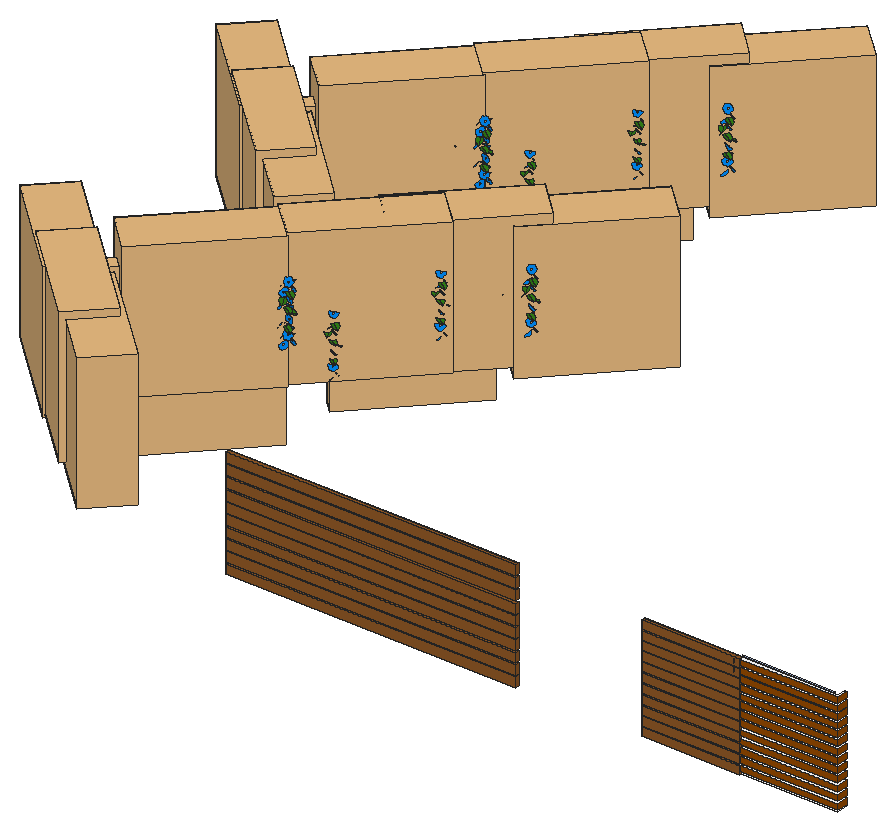
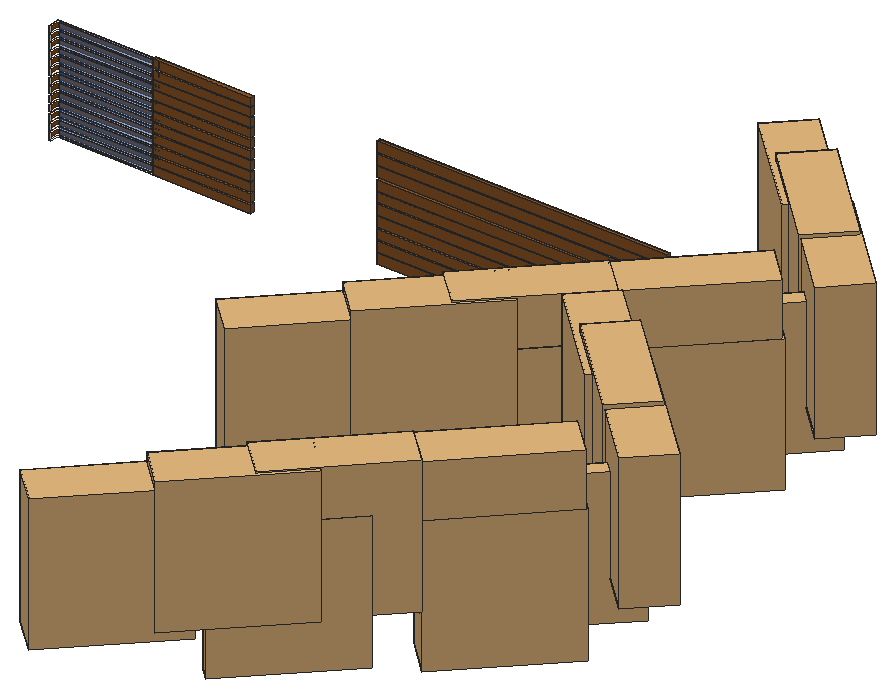
# SketchUp Ruby script. Lengths in inches.
U = 1.inch
M = Sketchup.active_model
def pt(a) = Geom::Point3d.new(a.map { |v| v * U })
def face(e, loops, mat)
  f = e.add_face(loops[0].map { |a| pt(a) })
  loops[1..].each { |l| e.add_face(l.map { |a| pt(a) }).erase! }
  f.material = f.back_material = mat if mat
  f
end
# faces: each face lists its corners as indices into pts; further lists are holes
def faces(e, pts, list, mat = nil) = list.each { |f| face(e, (f[0].is_a?(Array) ? f : [f]).map { |l| l.map { |i| pts[i] } }, mat) }
# xy, xz, yz: faces in a plane at the given z, y or x. An outline is a flat list of corners, or four numbers for a rectangle; further outlines are holes
def ring(l) = l.size == 4 ? [[l[0], l[1]], [l[2], l[1]], [l[2], l[3]], [l[0], l[3]]] : l.each_slice(2).to_a
def flat(e, list, mat, &to3) = list.each { |f| face(e, (f[0].is_a?(Array) ? f : [f]).map { |l| ring(l).map { |u, v| to3.(u, v) } }, mat) }
def xy(e, z, list, mat = nil) = flat(e, list, mat) { |x, y| [x, y, z] }
def xz(e, y, list, mat = nil) = flat(e, list, mat) { |x, z| [x, y, z] }
def yz(e, x, list, mat = nil) = flat(e, list, mat) { |y, z| [x, y, z] }
def lines(e, pts, list) = list.each { |a, b| e.add_line(pt(pts[a]), pt(pts[b])) }
# prism: a flat outline (further loops are holes) pulled along v
def prism(e, loops, v, mat = nil)
  f = face(e, loops, mat); d = Geom::Vector3d.new(v.map { |x| x * U })
  f.pushpull(f.normal.samedirection?(d) ? d.length : -d.length)
end
def box(e, o, s, mat = nil) = prism(e, [[o, [o[0] + s[0], o[1], o[2]], [o[0] + s[0], o[1] + s[1], o[2]], [o[0], o[1] + s[1], o[2]]]], [0, 0, s[2]], mat)
def at(x, y, z, deg = 0) = Geom::Transformation.translation(pt([x, y, z])) * Geom::Transformation.rotation(ORIGIN, Z_AXIS, deg.degrees)
def axes(o, x, y, z) = Geom::Transformation.new([*x, 0, *y, 0, *z, 0, *pt(o).to_a, 1])
def part(name) = M.definitions.add(name)
# library, detail: a bought-in or finely detailed component or shape, given as its bounding box
def library(name, o, s) = part(name).tap { |d| box(d.entities, o, s) }
def detail(e, o, s) = box(e.add_group.entities, o, s)
def put(e, d, t, mat = nil) = e.add_instance(d, t).tap { |i| i.material = mat if mat }
def group(e, t, mat = nil) = e.add_group.tap { |g| g.transformation = t; g.material = mat if mat }.entities
root = M.entities
M.materials.add("[Color C07]").color = [153, 76, 0]
M.materials.add("[Color M00]").color = [255, 255, 255]
M.materials.add("[Granite Tile]").color = [155, 148, 143]
M.materials.add("[Translucent Glass Blue]").color = [100, 149, 237]
M.materials["[Translucent Glass Blue]"].alpha = 0.5
M.materials.add("[Wood Floor Parquet]").color = [145, 89, 39]
M.materials.add("skp avat flo 1").color = [0, 129, 229]
M.materials.add("skp avat flo 2").color = [47, 120, 22]
c1 = part("Group\#24")
box(c1.entities,[0,-2.3125,0],[173.47,2.3125,5.79])
c2 = part("Group\#17")
box(c2.entities,[0,-2.125,0],[58.6875,4.9375,2.3125])
c3 = library("ruselia",[-5.83,-15.14,-32.53],[55.24,20.14,57.16])
c4 = part("Gruppe\#2")
xy(c4.entities,0,[[6.69,0,4.96,0.23,3.03,1.59,1.96,1.96,0.9,3.35,0.9,5.71,0,6.69,0.23,8.43,1.96,10,3.35,12.49,4.67,13.04,7.04,12.49,8.72,13.04,10.04,12.49,11.43,11.43,12.05,9.15,13.39,6.69,13.16,4.96,12.49,3.35,10.41,2.22,8.43,0.23]],"skp avat flo 1")
c5 = part("Gruppe\#12")
xy(c5.entities,0,[[1.18,0.5,1.36,0.52,1.52,0.59,1.67,0.7,1.77,0.84,1.84,1,1.87,1.18,1.84,1.36,1.77,1.52,1.67,1.67,1.52,1.77,1.36,1.84,1.18,1.87,1,1.84,0.84,1.77,0.7,1.67,0.59,1.52,0.52,1.36,0.5,1.18,0.52,1,0.59,0.84,0.7,0.7,0.84,0.59,1,0.52]])
c6 = part("f.st. wop plant 01 blüte")
put(c6.entities,c4,at(0,0,0))
put(c6.entities,c5,at(5.65,5.41,0.39))
c7 = part("Gruppe\#5")
xy(c7.entities,0.96,[[13.97,0.22,8.73,4.42,7.37,10.11,8.43,14.53,13.97,16.39]],"skp avat flo 2")
p = [[13.97,0.22,0.96],[13.97,16.39,0.96],[17.89,14.53,4.875],[18.64,10.11,5.625],[17.67,4.42,4.66]]
faces(c7.entities,p,[[0,1,2,3,4]],"skp avat flo 2")
c8 = part("f.st. wop plant 01 blatt")
put(c8.entities,c7,axes([0.99,0,4.74],[0.91566,0,-0.40195],[0,1,0],[0.40195,0,0.91566]))
c9 = part("Gruppe\#10")
put(c9.entities,c6,axes([4.61,0.45,57.14],[0.99373,-0.06775,-0.08889],[0.11172,0.62588,0.77188],[0.00335,-0.77697,0.62953]))
put(c9.entities,c6,axes([12.4,0.4,0.59],[0.70061,0.70799,-0.08889],[-0.40079,0.49353,0.77188],[0.59035,-0.50516,0.62953]))
put(c9.entities,c6,axes([24.4375,6.09,17.58],[-0.05734,0.99439,-0.08889],[-0.63495,0.03239,0.77188],[0.77043,0.1007,0.62953]))
put(c9.entities,c6,axes([1.11,8.09,13.25],[0.88983,-0.44754,-0.08889],[0.34553,0.53368,0.77188],[-0.298,-0.71756,0.62953]))
put(c9.entities,c6,axes([23.26,15,37.53],[-0.84836,0.52191,-0.08889],[-0.38985,-0.50222,0.77188],[0.35821,0.68948,0.62953]))
put(c9.entities,c6,axes([12.67,23.61,24.88],[-0.75852,-0.64555,-0.08889],[0.35717,-0.52596,0.77188],[-0.54504,0.55374,0.62953]))
put(c9.entities,c6,axes([20.43,22.9,81.42],[-0.98432,0.15238,-0.08889],[-0.16477,-0.61405,0.77188],[0.06303,0.77442,0.62953]))
put(c9.entities,c6,axes([1.76,2.9,29.21],[0.93833,-0.33412,-0.08889],[0.27691,0.5723,0.77188],[-0.20703,-0.74889,0.62953]))
put(c9.entities,c6,axes([13.59,0.5,77.09],[0.62412,0.77625,-0.08889],[-0.4494,0.44972,0.77188],[0.63915,-0.4418,0.62953]))
put(c9.entities,c6,axes([-1.26,15.51,69.79],[0.24265,-0.96603,-0.08889],[0.62977,0.08716,0.77188],[-0.73791,-0.24328,0.62953]))
put(c9.entities,c6,axes([22.04,17.92,65.46],[-0.95793,0.27287,-0.08889],[-0.2394,-0.58898,0.77188],[0.15827,0.76069,0.62953]))
put(c9.entities,c6,axes([9.51,23.35,52.81],[-0.55554,-0.82673,-0.08889],[0.48617,-0.40969,0.77188],[-0.67455,0.38559,0.62953]))
put(c9.entities,c6,axes([0.1875,18.97,41.86],[-0.02781,-0.99565,-0.08889],[0.62986,-0.08651,0.77188],[-0.77621,-0.03452,0.62953]))
put(c9.entities,c6,axes([24.98,7.4,94.08],[-0.15925,0.98323,-0.08889],[-0.63491,-0.03305,0.77188],[0.75599,0.17936,0.62953]))
put(c9.entities,c6,axes([21.5,21.98,4.93],[-0.96344,0.25275,-0.08889],[-0.22702,-0.59386,0.77188],[0.1423,0.76384,0.62953]))
put(c9.entities,c6,axes([1.57,6.98,89.75],[0.93112,-0.3537,-0.08889],[0.28884,0.56637,0.77188],[-0.22267,-0.74439,0.62953]))
put(c9.entities,c8,axes([9.37,32.32,90.95],[-0.51317,-0.65235,0],[0.5996,-0.47167,0.32697],[-0.25699,0.20216,0.76288]))
put(c9.entities,c8,axes([33.81,6.72,78.35],[-0.27992,0.78137,0],[-0.71819,-0.25729,0.32697],[0.30782,0.11027,0.76288]))
put(c9.entities,c8,axes([-9.46,14.86,61.47],[0.53029,-0.63851,0],[0.58688,0.4874,0.32697],[-0.25154,-0.2089,0.76288]))
put(c9.entities,c8,axes([21.49,-6.15,66.98],[0.2591,0.78852,0],[-0.72476,0.23815,0.32697],[0.31063,-0.10207,0.76288]))
put(c9.entities,c8,axes([32.03,5.27,54.38],[-0.36397,0.74594,0],[-0.68562,-0.33454,0.32697],[0.29386,0.14338,0.76288]))
put(c9.entities,c8,axes([30.63,20.6,49.31],[-0.77544,0.29596,0],[-0.27203,-0.71273,0.32697],[0.11659,0.30548,0.76288]))
put(c9.entities,c8,axes([32.03,5.27,27.16],[-0.36397,0.74594,0],[-0.68562,-0.33454,0.32697],[0.29386,0.14338,0.76288]))
put(c9.entities,c8,axes([17.4375,27.53,13.8125],[-0.76735,-0.23527,0.21148],[0.29408,-0.735,0.24937],[0.11659,0.30548,0.76288]))
put(c9.entities,c8,axes([-9.46,14.86,34.24],[0.53029,-0.63851,0],[0.58688,0.4874,0.32697],[-0.25154,-0.2089,0.76288]))
c10 = part("Gruppe\#9")
put(c10.entities,c6,axes([2.2,1.62,57.61],[0.97169,-0.0623,-0.22792],[0.22172,0.57378,0.78843],[0.08166,-0.81664,0.57134]))
put(c10.entities,c6,axes([-1.48,7.53,1.27],[0.68093,0.71536,-0.15682],[-0.22028,0.40428,0.88771],[0.69843,-0.56993,0.43287]))
put(c10.entities,c6,axes([13.97,11.34,15.86],[-0.0542,0.99797,0.03349],[-0.45869,-0.05467,0.88691],[0.88694,0.03271,0.46072]))
put(c10.entities,c6,axes([-9.71,13.74,16.77],[0.84218,-0.4326,-0.32186],[0.5102,0.4462,0.73526],[-0.17446,-0.78343,0.59649]))
put(c10.entities,c6,axes([17.17,17.99,36.46],[-0.83727,0.52624,0.14846],[-0.23006,-0.58536,0.77745],[0.49603,0.61679,0.61117]))
put(c10.entities,c6,axes([4.35,27.92,27.32],[-0.77345,-0.63385,0.00301],[0.4998,-0.60694,0.61792],[-0.38984,0.47943,0.78623]))
put(c10.entities,c6,axes([20.43,22.9,81.42],[-0.98432,0.15238,-0.08889],[-0.16477,-0.61405,0.77188],[0.06303,0.77442,0.62953]))
put(c10.entities,c6,axes([-5.84,6.82,31.58],[0.89192,-0.31974,-0.31975],[0.44391,0.4844,0.75386],[-0.08616,-0.81432,0.57398]))
put(c10.entities,c6,axes([13.59,0.5,77.09],[0.62412,0.77625,-0.08889],[-0.4494,0.44972,0.77188],[0.63915,-0.4418,0.62953]))
put(c10.entities,c6,axes([-1.26,15.51,69.79],[0.24265,-0.96603,-0.08889],[0.62977,0.08716,0.77188],[-0.73791,-0.24328,0.62953]))
put(c10.entities,c6,axes([20.77,18.5,64.59],[-0.95848,0.27864,0.06062],[-0.13765,-0.63827,0.75741],[0.24973,0.71762,0.65012]))
put(c10.entities,c6,axes([6.6875,24.75,54.15],[-0.57029,-0.8188,-0.06577],[0.58283,-0.45976,0.67002],[-0.57885,0.34377,0.73942]))
put(c10.entities,c6,axes([-4.08,21.11,44.3125],[-0.04911,-0.98765,-0.14878],[0.72825,-0.13735,0.67141],[-0.68355,-0.07538,0.726]))
put(c10.entities,c6,axes([24.98,7.4,94.08],[-0.15925,0.98323,-0.08889],[-0.63491,-0.03305,0.77188],[0.75599,0.17936,0.62953]))
put(c10.entities,c6,axes([8.77,28.52,5.9],[-0.95532,0.25842,0.14346],[-0.07274,-0.676,0.7333],[0.28648,0.6901,0.6646]))
put(c10.entities,c6,axes([1.57,6.98,89.75],[0.93112,-0.3537,-0.08889],[0.28884,0.56637,0.77188],[-0.22267,-0.74439,0.62953]))
put(c10.entities,c8,axes([9.37,32.32,90.95],[-0.51317,-0.65235,0],[0.5996,-0.47167,0.32697],[-0.25699,0.20216,0.76288]))
put(c10.entities,c8,axes([33.81,6.72,78.35],[-0.27992,0.78137,0],[-0.71819,-0.25729,0.32697],[0.30782,0.11027,0.76288]))
put(c10.entities,c8,axes([-11.01,15.72,64.74],[0.51926,-0.63742,-0.11388],[0.63054,0.46456,0.27478],[-0.14729,-0.25842,0.77487]))
put(c10.entities,c8,axes([20.21,-5.625,64.6],[0.26417,0.78668,0.01588],[-0.67119,0.21655,0.43762],[0.41063,-0.15212,0.70508]))
put(c10.entities,c8,axes([29.04,6.59,51.45],[-0.35348,0.74452,0.09816],[-0.63785,-0.35493,0.39506],[0.39635,0.09281,0.72332]))
put(c10.entities,c8,axes([27.11,22.23,47.625],[-0.76537,0.29574,0.12508],[-0.23173,-0.73252,0.31403],[0.22228,0.25465,0.75805]))
put(c10.entities,c8,axes([23.375,9.49,23.48],[-0.34051,0.7404,0.15735],[-0.60881,-0.37042,0.42548],[0.44978,0.05914,0.69506]))
put(c10.entities,c8,axes([6.77,33.04,15.99],[-0.71083,-0.25923,0.3412],[0.32455,-0.75723,0.10082],[0.2798,0.21977,0.74988]))
put(c10.entities,c8,axes([-15.51,18.125,40.12],[0.50532,-0.63318,-0.18065],[0.65217,0.44994,0.24724],[-0.09068,-0.29247,0.77145]))
c11 = part("Gruppe\#11")
put(c11.entities,c6,axes([4.61,0.45,57.14],[0.99373,-0.06775,-0.08889],[0.11172,0.62588,0.77188],[0.00335,-0.77697,0.62953]))
put(c11.entities,c6,axes([12.4,0.4,0.59],[0.70061,0.70799,-0.08889],[-0.40079,0.49353,0.77188],[0.59035,-0.50516,0.62953]))
put(c11.entities,c6,axes([24.4375,6.09,17.58],[-0.05734,0.99439,-0.08889],[-0.63495,0.03239,0.77188],[0.77043,0.1007,0.62953]))
put(c11.entities,c6,axes([1.11,8.09,13.25],[0.88983,-0.44754,-0.08889],[0.34553,0.53368,0.77188],[-0.298,-0.71756,0.62953]))
put(c11.entities,c6,axes([23.26,15,37.53],[-0.84836,0.52191,-0.08889],[-0.38985,-0.50222,0.77188],[0.35821,0.68948,0.62953]))
put(c11.entities,c6,axes([12.67,23.61,24.88],[-0.75852,-0.64555,-0.08889],[0.35717,-0.52596,0.77188],[-0.54504,0.55374,0.62953]))
put(c11.entities,c6,axes([20.43,22.9,81.42],[-0.98432,0.15238,-0.08889],[-0.16477,-0.61405,0.77188],[0.06303,0.77442,0.62953]))
put(c11.entities,c6,axes([1.76,2.9,29.21],[0.93833,-0.33412,-0.08889],[0.27691,0.5723,0.77188],[-0.20703,-0.74889,0.62953]))
put(c11.entities,c6,axes([13.59,0.5,77.09],[0.62412,0.77625,-0.08889],[-0.4494,0.44972,0.77188],[0.63915,-0.4418,0.62953]))
put(c11.entities,c6,axes([-1.26,15.51,69.79],[0.24265,-0.96603,-0.08889],[0.62977,0.08716,0.77188],[-0.73791,-0.24328,0.62953]))
put(c11.entities,c6,axes([22.04,17.92,65.46],[-0.95793,0.27287,-0.08889],[-0.2394,-0.58898,0.77188],[0.15827,0.76069,0.62953]))
put(c11.entities,c6,axes([9.51,23.35,52.81],[-0.55554,-0.82673,-0.08889],[0.48617,-0.40969,0.77188],[-0.67455,0.38559,0.62953]))
put(c11.entities,c6,axes([0.1875,18.97,41.86],[-0.02781,-0.99565,-0.08889],[0.62986,-0.08651,0.77188],[-0.77621,-0.03452,0.62953]))
put(c11.entities,c6,axes([24.98,7.4,94.08],[-0.15925,0.98323,-0.08889],[-0.63491,-0.03305,0.77188],[0.75599,0.17936,0.62953]))
put(c11.entities,c6,axes([21.5,21.98,4.93],[-0.96344,0.25275,-0.08889],[-0.22702,-0.59386,0.77188],[0.1423,0.76384,0.62953]))
put(c11.entities,c6,axes([1.57,6.98,89.75],[0.93112,-0.3537,-0.08889],[0.28884,0.56637,0.77188],[-0.22267,-0.74439,0.62953]))
put(c11.entities,c8,axes([9.37,32.32,90.95],[-0.51317,-0.65235,0],[0.5996,-0.47167,0.32697],[-0.25699,0.20216,0.76288]))
put(c11.entities,c8,axes([33.81,6.72,78.35],[-0.27992,0.78137,0],[-0.71819,-0.25729,0.32697],[0.30782,0.11027,0.76288]))
put(c11.entities,c8,axes([-9.46,14.86,61.47],[0.53029,-0.63851,0],[0.58688,0.4874,0.32697],[-0.25154,-0.2089,0.76288]))
put(c11.entities,c8,axes([21.49,-6.15,66.98],[0.2591,0.78852,0],[-0.72476,0.23815,0.32697],[0.31063,-0.10207,0.76288]))
put(c11.entities,c8,axes([32.03,5.27,54.38],[-0.36397,0.74594,0],[-0.68562,-0.33454,0.32697],[0.29386,0.14338,0.76288]))
put(c11.entities,c8,axes([30.63,20.6,49.31],[-0.77544,0.29596,0],[-0.27203,-0.71273,0.32697],[0.11659,0.30548,0.76288]))
put(c11.entities,c8,axes([32.03,5.27,27.16],[-0.36397,0.74594,0],[-0.68562,-0.33454,0.32697],[0.29386,0.14338,0.76288]))
put(c11.entities,c8,axes([17.4375,27.53,13.8125],[-0.76735,-0.23527,0.21148],[0.29408,-0.735,0.24937],[0.11659,0.30548,0.76288]))
put(c11.entities,c8,axes([-9.46,14.86,34.24],[0.53029,-0.63851,0],[0.58688,0.4874,0.32697],[-0.25154,-0.2089,0.76288]))
c12 = part("Gruppe\#8")
put(c12.entities,c6,axes([2.26,1.13,59.39],[0.92531,-0.05375,-0.37538],[0.3384,0.56379,0.75341],[0.17114,-0.82417,0.53987]))
put(c12.entities,c6,axes([-9.39,6.25,4.33],[0.64151,0.72107,-0.26176],[-0.09814,0.41557,0.90425],[0.76081,-0.5544,0.33735]))
put(c12.entities,c6,axes([7.9,10.48,16.53],[-0.06325,0.99763,0.02691],[-0.32763,-0.04623,0.94367],[0.94269,0.05087,0.32978]))
put(c12.entities,c6,axes([-15.4375,12.6,20.76],[0.79424,-0.42729,-0.43198],[0.60271,0.46401,0.64918],[-0.07695,-0.77596,0.62607]))
put(c12.entities,c6,axes([13.9,17.49,36.37],[-0.81529,0.51823,0.25834],[-0.1092,-0.57574,0.81031],[0.56867,0.63242,0.52599]))
put(c12.entities,c6,axes([-0.23,27.12,29.01],[-0.75604,-0.64315,0.1215],[0.59094,-0.59091,0.5492],[-0.28142,0.48702,0.82681]))
put(c12.entities,c6,axes([20.43,22.9,81.42],[-0.98432,0.15238,-0.08889],[-0.16477,-0.61405,0.77188],[0.06303,0.77442,0.62953]))
put(c12.entities,c6,axes([-9.41,5.97,34.96],[0.84215,-0.31382,-0.43852],[0.53918,0.50168,0.67646],[0.00771,-0.80612,0.5917]))
put(c12.entities,c6,axes([13.59,0.5,77.09],[0.62412,0.77625,-0.08889],[-0.4494,0.44972,0.77188],[0.63915,-0.4418,0.62953]))
put(c12.entities,c6,axes([-1.26,15.51,69.79],[0.24265,-0.96603,-0.08889],[0.62977,0.08716,0.77188],[-0.73791,-0.24328,0.62953]))
put(c12.entities,c6,axes([22.04,17.92,65.46],[-0.95793,0.27287,-0.08889],[-0.2394,-0.58898,0.77188],[0.15827,0.76069,0.62953]))
put(c12.entities,c6,axes([6.08,24.33,55.62],[-0.57097,-0.82091,0.01051],[0.68037,-0.46598,0.56565],[-0.45945,0.33012,0.82458]))
put(c12.entities,c6,axes([-6.06,20.77,47.51],[-0.06819,-0.9857,-0.15407],[0.82323,-0.14283,0.54945],[-0.56361,-0.08937,0.8212]))
put(c12.entities,c6,axes([24.98,7.4,94.08],[-0.15925,0.98323,-0.08889],[-0.63491,-0.03305,0.77188],[0.75599,0.17936,0.62953]))
put(c12.entities,c6,axes([1.11,27.4375,7.17],[-0.92899,0.24893,0.27387],[0.04156,-0.66514,0.74556],[0.36776,0.70401,0.60756]))
put(c12.entities,c6,axes([1.57,6.98,89.75],[0.93112,-0.3537,-0.08889],[0.28884,0.56637,0.77188],[-0.22267,-0.74439,0.62953]))
put(c12.entities,c8,axes([9.37,32.32,90.95],[-0.51317,-0.65235,0],[0.5996,-0.47167,0.32697],[-0.25699,0.20216,0.76288]))
put(c12.entities,c8,axes([33.81,6.72,78.35],[-0.27992,0.78137,0],[-0.71819,-0.25729,0.32697],[0.30782,0.11027,0.76288]))
put(c12.entities,c8,axes([-9.74,15.05,68.68],[0.49765,-0.63289,-0.20172],[0.66377,0.46408,0.1815],[-0.02561,-0.27014,0.78439]))
put(c12.entities,c8,axes([21.49,-6.15,66.98],[0.2591,0.78852,0],[-0.72476,0.23815,0.32697],[0.31063,-0.10207,0.76288]))
put(c12.entities,c8,axes([27.8125,6.34,49.26],[-0.33661,0.74111,0.1623],[-0.5684,-0.36396,0.48306],[0.5025,0.08476,0.65514]))
put(c12.entities,c8,axes([25.26,22.01,46],[-0.73801,0.28975,0.24554],[-0.17833,-0.73814,0.33502],[0.33532,0.24514,0.71859]))
put(c12.entities,c8,axes([18.32,8.86,22.77],[-0.32541,0.73857,0.19371],[-0.53703,-0.37106,0.51265],[0.54278,0.07565,0.62335]))
put(c12.entities,c8,axes([0.49,32.09,17.38],[-0.65154,-0.26248,0.44214],[0.34641,-0.75151,0.06433],[0.37999,0.23503,0.69948]))
put(c12.entities,c8,axes([-17.94,17.29,44.63],[0.48369,-0.62973,-0.24163],[0.67408,0.46176,0.14595],[0.0237,-0.2813,0.78052]))
c13 = part("f.st. wop plant 01")
put(c13.entities,c9,at(39.14,64.09,18.66,-141.2))
put(c13.entities,c10,axes([53.54,120.93,12.24],[-0.61849,0.75929,0.20233],[-0.78178,-0.62056,-0.06099],[0.07925,-0.1959,0.97742]))
put(c13.entities,c11,at(82.26,36.89,18.66))
put(c13.entities,c12,axes([72.55,-5.87,29.3],[0.62579,-0.70508,0.33355],[0.76326,0.64164,-0.07566],[-0.16067,0.30193,0.93969]))
c14 = part("World of Pandora - tree 01")
put(c14.entities,c13,at(57.06,8.63,0))
xy(root,151.34,[[561.375,211.8125,623.5625,211.8125,623.5625,218.625,622.25,218.625,622.25,213.625,561.375,213.625]],"[Color M00]")
xy(root,152.15,[[561.375,211.8125,561.375,213.625,622.25,213.625,622.25,218.625,623.5625,218.625,623.5625,211.8125]],"[Color M00]")
xy(root,155.71,[[561.375,211.8125,623.5625,211.8125,623.5625,218.625,622.25,218.625,622.25,213.625,561.375,213.625]],"[Color M00]")
xy(root,156.9,[[561.375,211.8125,561.375,213.625,622.25,213.625,622.25,218.625,623.5625,218.625,623.5625,211.8125]],"[Color M00]")
xy(root,160.46,[[561.375,211.8125,623.5625,211.8125,623.5625,218.625,622.25,218.625,622.25,213.625,561.375,213.625]],"[Color M00]")
xy(root,161.71,[[561.375,211.8125,561.375,213.625,622.25,213.625,622.25,218.625,623.5625,218.625,623.5625,211.8125]],"[Color M00]")
xy(root,165.27,[[561.375,211.8125,623.5625,211.8125,623.5625,218.625,622.25,218.625,622.25,213.625,561.375,213.625]],"[Color M00]")
xy(root,166.77,[[561.375,211.8125,561.375,213.625,622.25,213.625,622.25,218.625,623.5625,218.625,623.5625,211.8125]],"[Color M00]")
xy(root,170.34,[[561.375,211.8125,623.5625,211.8125,623.5625,218.625,622.25,218.625,622.25,213.625,561.375,213.625]],"[Color M00]")
xy(root,171.65,[[561.375,211.8125,561.375,213.625,622.25,213.625,622.25,218.625,623.5625,218.625,623.5625,211.8125]],"[Color M00]")
xy(root,175.21,[[561.375,211.8125,623.5625,211.8125,623.5625,218.625,622.25,218.625,622.25,213.625,561.375,213.625]],"[Color M00]")
xy(root,176.52,[[561.375,211.8125,561.375,213.625,622.25,213.625,622.25,218.625,623.5625,218.625,623.5625,211.8125]],"[Color M00]")
xy(root,180.09,[[561.375,211.8125,623.5625,211.8125,623.5625,218.625,622.25,218.625,622.25,213.625,561.375,213.625]],"[Color M00]")
xy(root,181.34,[[561.375,211.8125,561.375,213.625,622.25,213.625,622.25,218.625,623.5625,218.625,623.5625,211.8125]],"[Color M00]")
xy(root,184.9,[[561.375,211.8125,623.5625,211.8125,623.5625,218.625,622.25,218.625,622.25,213.625,561.375,213.625]],"[Color M00]")
xy(root,186.34,[[561.375,211.8125,561.375,213.625,622.25,213.625,622.25,218.625,623.5625,218.625,623.5625,211.8125]],"[Color M00]")
xy(root,189.9,[[561.375,211.8125,623.5625,211.8125,623.5625,218.625,622.25,218.625,622.25,213.625,561.375,213.625]],"[Color M00]")
xy(root,190.96,[[561.375,211.8125,561.375,213.625,622.25,213.625,622.25,218.625,623.5625,218.625,623.5625,211.8125]],"[Color M00]")
xy(root,194.52,[[561.375,211.8125,623.5625,211.8125,623.5625,218.625,622.25,218.625,622.25,213.625,561.375,213.625]],"[Color M00]")
xy(root,195.52,[[561.375,211.8125,561.375,213.625,622.25,213.625,622.25,218.625,623.5625,218.625,623.5625,211.8125]],"[Color M00]")
xy(root,199.09,[[561.375,211.8125,623.5625,211.8125,623.5625,218.625,622.25,218.625,622.25,213.625,561.375,213.625]],"[Color M00]")
xy(root,200.21,[[561.375,211.8125,561.375,213.625,622.25,213.625,622.25,218.625,623.5625,218.625,623.5625,211.8125]],"[Color M00]")
xy(root,203.77,[[561.375,211.8125,623.5625,211.8125,623.5625,218.625,622.25,218.625,622.25,213.625,561.375,213.625]],"[Color M00]")
xy(root,204.71,[[561.375,211.8125,561.375,213.625,622.25,213.625,622.25,218.625,623.5625,218.625,623.5625,211.8125]],"[Color M00]")
xy(root,208.27,[[561.375,211.8125,623.5625,211.8125,623.5625,218.625,622.25,218.625,622.25,213.625,561.375,213.625]],"[Color M00]")
xy(root,209.21,[[561.375,211.8125,561.375,213.625,622.25,213.625,622.25,218.625,623.5625,218.625,623.5625,211.8125]],"[Color M00]")
xy(root,212.77,[[561.375,211.8125,623.5625,211.8125,623.5625,218.625,622.25,218.625,622.25,213.625,561.375,213.625]],"[Color M00]")
xz(root,211.8125,[[561.375,152.15,623.5625,155.71],[561.375,156.9,623.5625,160.46],[561.375,161.71,623.5625,165.27],[561.375,166.77,623.5625,170.34],[561.375,171.65,623.5625,175.21],
  [561.375,176.52,623.5625,180.09],[561.375,181.34,623.5625,184.9],[561.375,186.34,623.5625,189.9],[561.375,190.96,623.5625,194.52],[561.375,195.52,623.5625,199.09],
  [561.375,200.21,623.5625,203.77],[561.375,204.71,623.5625,208.27],[561.375,209.21,623.5625,212.77]],"[Color C07]")
xz(root,213.625,[[561.375,204.71,564.8125,208.27],[561.375,209.21,564.8125,212.77]],"[Color M00]")
xz(root,213.625,[[564.8125,151.34,620.9375,152.15],[564.8125,152.15,620.9375,155.71],[564.8125,155.71,620.9375,156.9],[564.8125,156.9,620.9375,160.46],[564.8125,160.46,620.9375,161.71],
  [564.8125,161.71,620.9375,165.27],[564.8125,165.27,620.9375,166.77],[564.8125,166.77,620.9375,170.34],[564.8125,170.34,620.9375,171.65],[564.8125,171.65,620.9375,175.21],
  [564.8125,175.21,620.9375,176.52],[564.8125,176.52,620.9375,180.09],[564.8125,180.09,620.9375,181.34],[564.8125,181.34,620.9375,184.9],[564.8125,184.9,620.9375,186.34],
  [564.8125,186.34,620.9375,189.9],[564.8125,189.9,620.9375,190.96],[564.8125,190.96,620.9375,194.52],[564.8125,194.52,620.9375,195.52],[564.8125,195.52,620.9375,199.09],
  [564.8125,199.09,620.9375,200.21],[564.8125,200.21,620.9375,203.77],[564.8125,203.77,620.9375,204.71],[564.8125,204.71,620.9375,208.27],[564.8125,208.27,620.9375,209.21],
  [564.8125,209.21,620.9375,212.77],[564.8125,212.77,620.9375,213.84]],"[Translucent Glass Blue]")
xz(root,218.625,[[622.25,152.15,623.5625,155.71],[622.25,156.9,623.5625,160.46],[622.25,161.71,623.5625,165.27],[622.25,166.77,623.5625,170.34],[622.25,171.65,623.5625,175.21],
  [622.25,176.52,623.5625,180.09],[622.25,181.34,623.5625,184.9],[622.25,186.34,623.5625,189.9],[622.25,190.96,623.5625,194.52],[622.25,195.52,623.5625,199.09],
  [622.25,200.21,623.5625,203.77],[622.25,204.71,623.5625,208.27],[622.25,209.21,623.5625,212.77]],"[Color M00]")
yz(root,561.375,[[211.8125,204.71,213.625,208.27],[211.8125,209.21,213.625,212.77]],"[Color M00]")
yz(root,623.5625,[[211.8125,152.15,218.625,155.71],[211.8125,156.9,218.625,160.46],[211.8125,161.71,218.625,165.27],[211.8125,166.77,218.625,170.34],[211.8125,171.65,218.625,175.21],
  [211.8125,176.52,218.625,180.09],[211.8125,181.34,218.625,184.9],[211.8125,186.34,218.625,189.9],[211.8125,190.96,218.625,194.52],[211.8125,195.52,218.625,199.09],
  [211.8125,200.21,218.625,203.77],[211.8125,204.71,218.625,208.27],[211.8125,209.21,218.625,212.77]],"[Color C07]")
put(root,c1,at(257.3125,213.625,150.3125),"[Wood Floor Parquet]")
put(root,c2,axes([506.125,213.625,152.89],[1,0,0],[0,0,1],[0,-1,0]),"[Wood Floor Parquet]")
put(root,c2,axes([506.125,213.625,158.64],[1,0,0],[0,0,1],[0,-1,0]),"[Wood Floor Parquet]")
put(root,c3,axes([173.95,492.49,202.7],[-0.97449,-1.03284,0],[1.03284,-0.97449,0],[0,0,1.42]),"[Granite Tile]")
put(root,c1,at(257.3125,213.625,156.875),"[Wood Floor Parquet]")
put(root,c3,axes([201.01,311.54,205.34],[-0.97449,-1.03284,0],[1.03284,-0.97449,0],[0,0,1.42]),"[Granite Tile]")
put(root,c3,axes([232.89,577.43,207.53],[-0.97449,-1.03284,0],[0.34084,-0.32158,0],[0,0,1.42]),"[Granite Tile]")
put(root,c2,axes([506.125,213.625,164.39],[1,0,0],[0,0,1],[0,-1,0]),"[Wood Floor Parquet]")
put(root,c1,at(257.3125,213.625,163.5),"[Wood Floor Parquet]")
put(root,c3,axes([259.94,396.48,210.16],[-0.97449,-1.03284,0],[0.34084,-0.32158,0],[0,0,1.42]),"[Granite Tile]")
put(root,c2,axes([506.125,213.625,170.2],[1,0,0],[0,0,1],[0,-1,0]),"[Wood Floor Parquet]")
put(root,c1,at(257.3125,213.625,170.1875),"[Wood Floor Parquet]")
put(root,c3,axes([129.57,454.6,217.3],[-0.57495,-0.60938,0],[0.34084,-0.32158,0],[0,0,1.42]),"[Granite Tile]")
put(root,c3,axes([156.63,273.65,219.93],[-0.57495,-0.60938,0],[0.34084,-0.32158,0],[0,0,1.42]),"[Granite Tile]")
put(root,c2,axes([506.125,213.625,176.08],[1,0,0],[0,0,1],[0,-1,0]),"[Wood Floor Parquet]")
put(root,c1,at(257.3125,213.625,176.75),"[Wood Floor Parquet]")
put(root,c2,axes([506.125,213.625,181.95],[1,0,0],[0,0,1],[0,-1,0]),"[Wood Floor Parquet]")
put(root,c3,axes([300.96,628.66,229.43],[-0.97449,-1.03284,0],[1.03284,-0.97449,0],[0,0,1.42]),"[Granite Tile]")
put(root,c1,at(257.3125,213.625,183.3125),"[Wood Floor Parquet]")
put(root,c14,axes([142.83,533.99,182.55],[0.26912,-0.25392,0],[0.25392,0.26912,0],[0,0,0.37]),"[Granite Tile]")
put(root,c2,axes([506.125,213.625,187.83],[1,0,0],[0,0,1],[0,-1,0]),"[Wood Floor Parquet]")
put(root,c3,axes([328.01,447.71,232.06],[-0.97449,-1.03284,0],[1.03284,-0.97449,0],[0,0,1.42]),"[Granite Tile]")
put(root,c14,axes([169.88,353.04,185.1875],[0.26912,-0.25392,0],[0.25392,0.26912,0],[0,0,0.37]),"[Granite Tile]")
put(root,c3,axes([175.09,492.96,234.27],[-0.97449,-1.03284,0],[1.03284,-0.97449,0],[0,0,1.42]),"[Granite Tile]")
put(root,c3,axes([259.1,586.19,234.75],[-0.97449,-1.03284,0],[1.03284,-0.97449,0],[0,0,1.42]),"[Granite Tile]")
put(root,c3,axes([227.98,549.84,235.2],[-0.97449,-1.03284,0],[1.03284,-0.97449,0],[0,0,1.42]),"[Granite Tile]")
put(root,c1,at(257.3125,213.625,189.66),"[Wood Floor Parquet]")
put(root,c3,axes([202.15,312.01,236.91],[-0.97449,-1.03284,0],[1.03284,-0.97449,0],[0,0,1.42]),"[Granite Tile]")
put(root,c3,axes([286.15,405.25,237.39],[-0.97449,-1.03284,0],[1.03284,-0.97449,0],[0,0,1.42]),"[Granite Tile]")
put(root,c2,axes([506.125,213.625,193.58],[1,0,0],[0,0,1],[0,-1,0]),"[Wood Floor Parquet]")
put(root,c3,axes([255.04,368.89,237.83],[-0.97449,-1.03284,0],[1.03284,-0.97449,0],[0,0,1.42]),"[Granite Tile]")
put(root,c3,axes([151.37,397.625,239.72],[1.03284,-0.97449,0],[0.97449,1.03284,0],[0,0,1.42]),"[Granite Tile]")
put(root,c3,axes([87.03,452.6,241.89],[1.03284,-0.97449,0],[0.97449,1.03284,0],[0,0,1.42]),"[Granite Tile]")
put(root,c3,axes([178.43,216.68,242.36],[1.03284,-0.97449,0],[0.97449,1.03284,0],[0,0,1.42]),"[Granite Tile]")
put(root,c1,at(257.3125,213.625,196.85),"[Wood Floor Parquet]")
put(root,c2,axes([506.125,213.625,199.14],[1,0,0],[0,0,1],[0,-1,0]),"[Wood Floor Parquet]")
put(root,c3,axes([122.22,420.65,243.87],[1.03284,-0.97449,0],[0.97449,1.03284,0],[0,0,1.42]),"[Granite Tile]")
put(root,c3,axes([114.09,271.65,244.52],[1.03284,-0.97449,0],[0.97449,1.03284,0],[0,0,1.42]),"[Granite Tile]")
put(root,c3,axes([149.28,239.7,246.5],[1.03284,-0.97449,0],[0.97449,1.03284,0],[0,0,1.42]),"[Granite Tile]")
put(root,c14,axes([207.08,602.1,198.79],[0.26912,-0.25392,0],[0.25392,0.26912,0],[0,0,0.37]),"[Granite Tile]")
put(root,c2,axes([506.125,213.625,204.7],[1,0,0],[0,0,1],[0,-1,0]),"[Wood Floor Parquet]")
put(root,c14,axes([177.7,570.95,200.31],[0.26912,-0.25392,0],[0.25392,0.26912,0],[0,0,0.37]),"[Granite Tile]")
put(root,c1,at(257.3125,213.625,203.6),"[Wood Floor Parquet]")
put(root,c14,axes([234.14,421.15,201.43],[0.26912,-0.25392,0],[0.25392,0.26912,0],[0,0,0.37]),"[Granite Tile]")
put(root,c14,axes([130.3,515.87,202.89],[0.26912,-0.25392,0],[0.25392,0.26912,0],[0,0,0.37]),"[Granite Tile]")
put(root,c14,axes([204.75,390,202.94],[0.26912,-0.25392,0],[0.25392,0.26912,0],[0,0,0.37]),"[Granite Tile]")
put(root,c14,axes([157.36,334.92,205.52],[0.26912,-0.25392,0],[0.25392,0.26912,0],[0,0,0.37]),"[Granite Tile]")
put(root,c2,axes([506.125,213.625,210.33],[1,0,0],[0,0,1],[0,-1,0]),"[Wood Floor Parquet]")
put(root,c1,at(257.3125,213.625,210.35),"[Wood Floor Parquet]")
